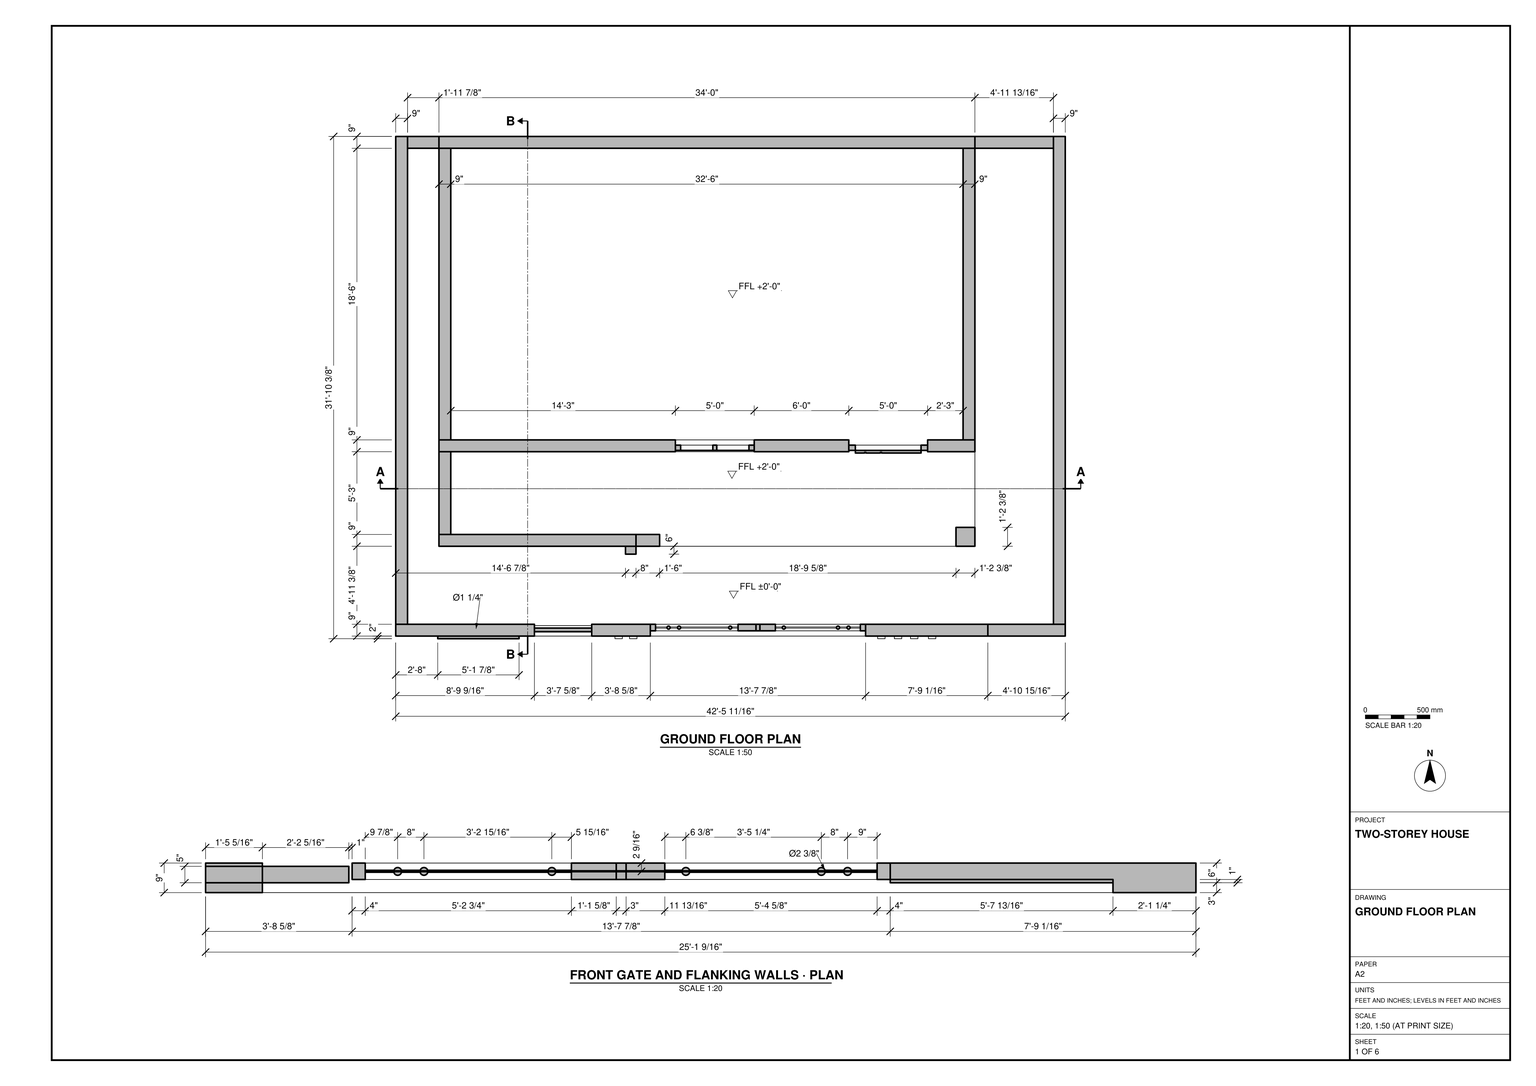
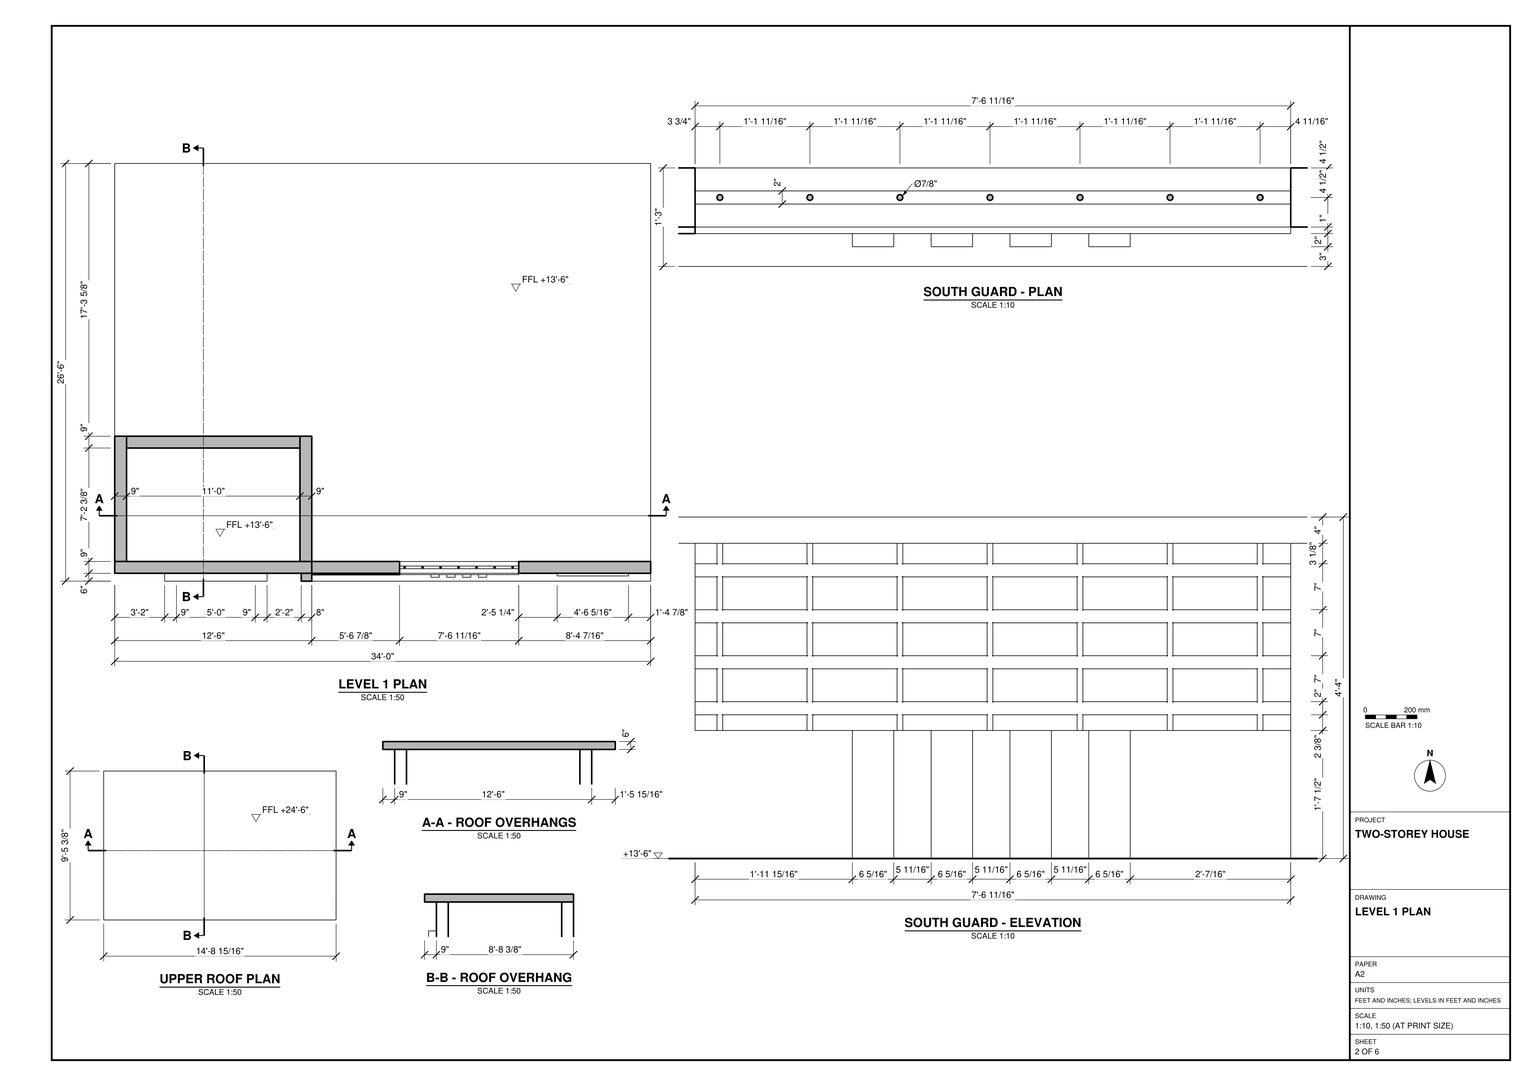
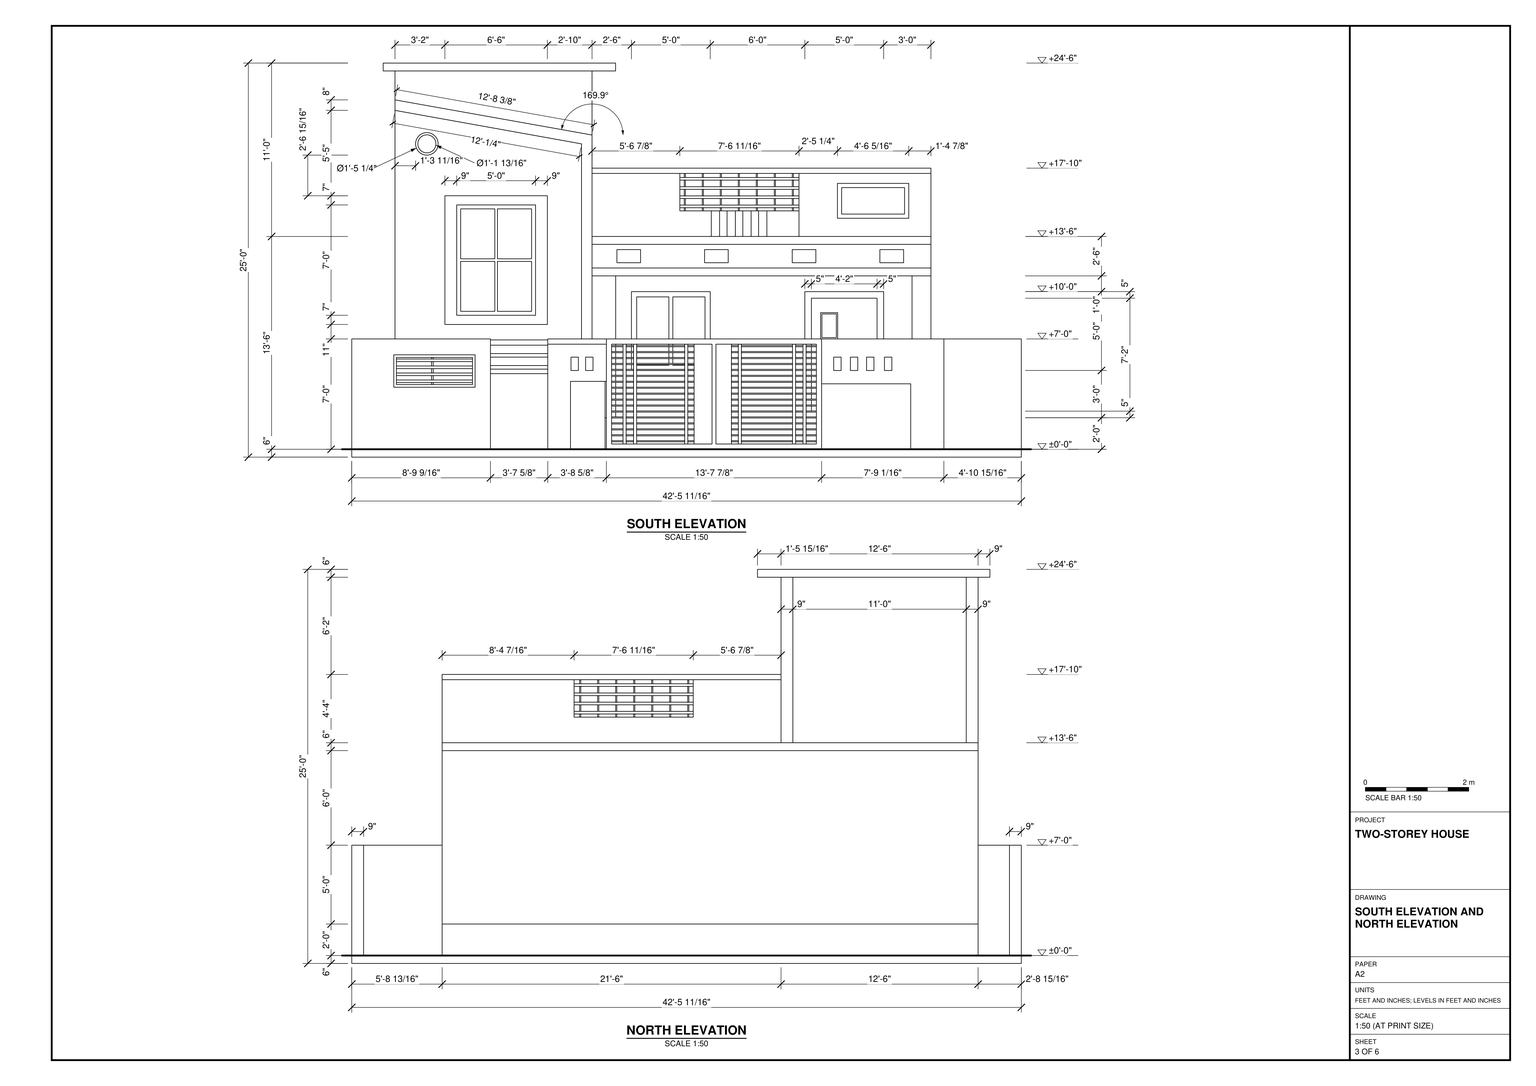
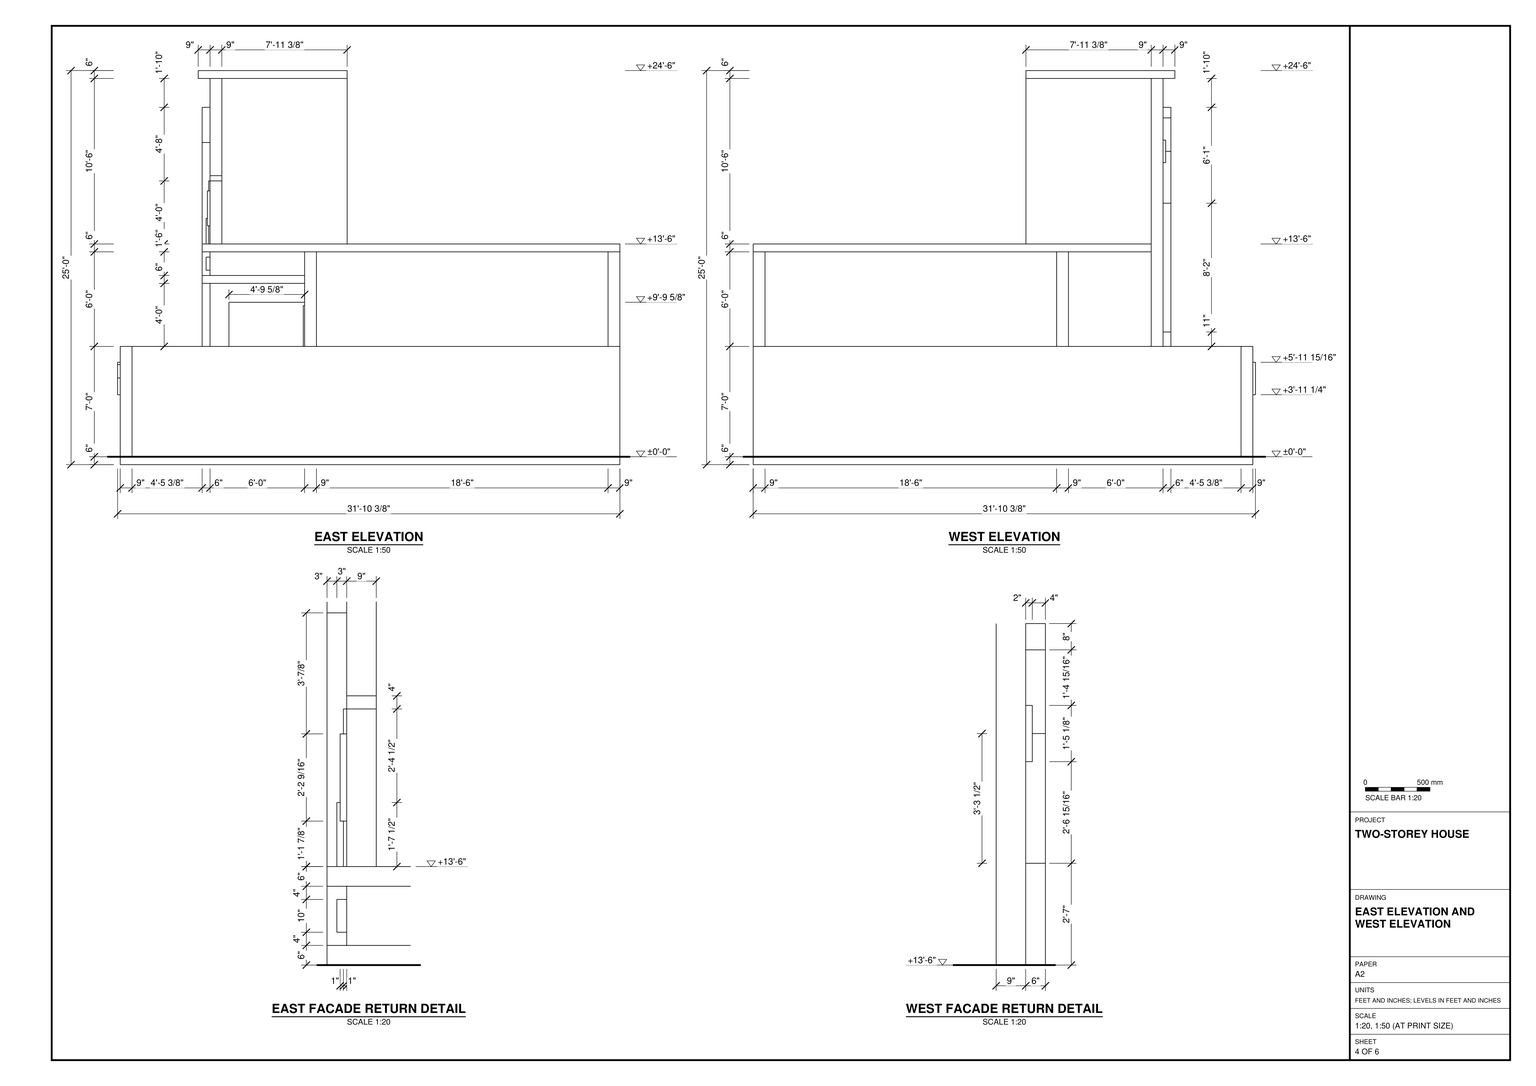
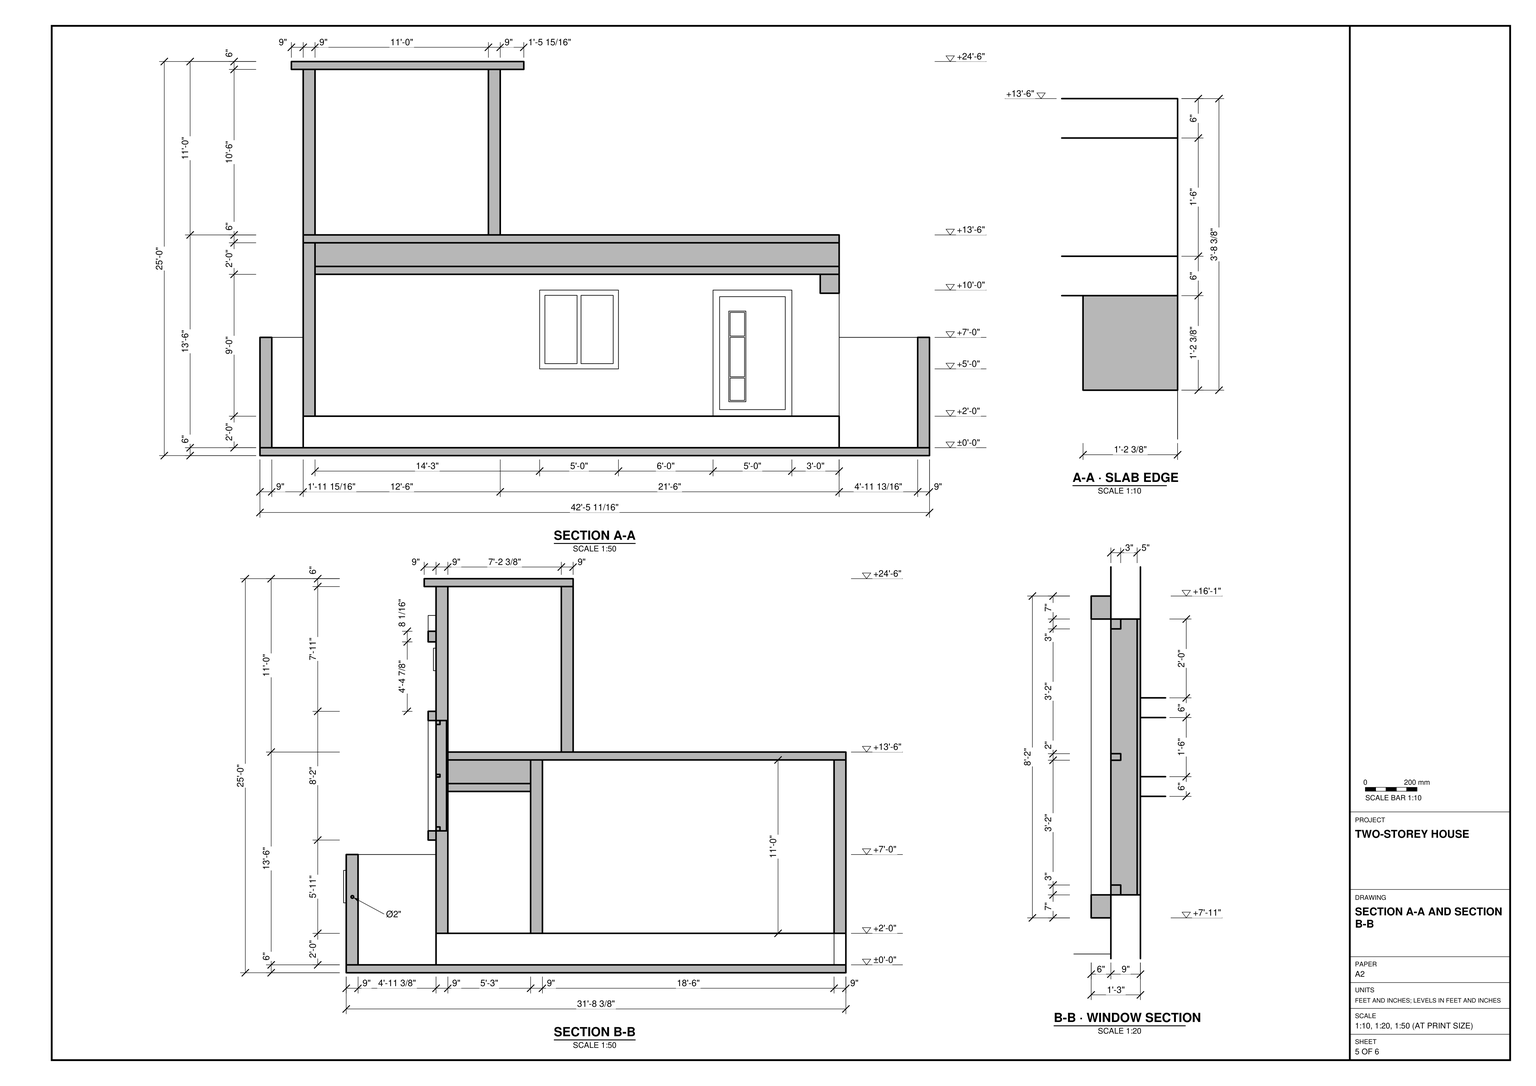
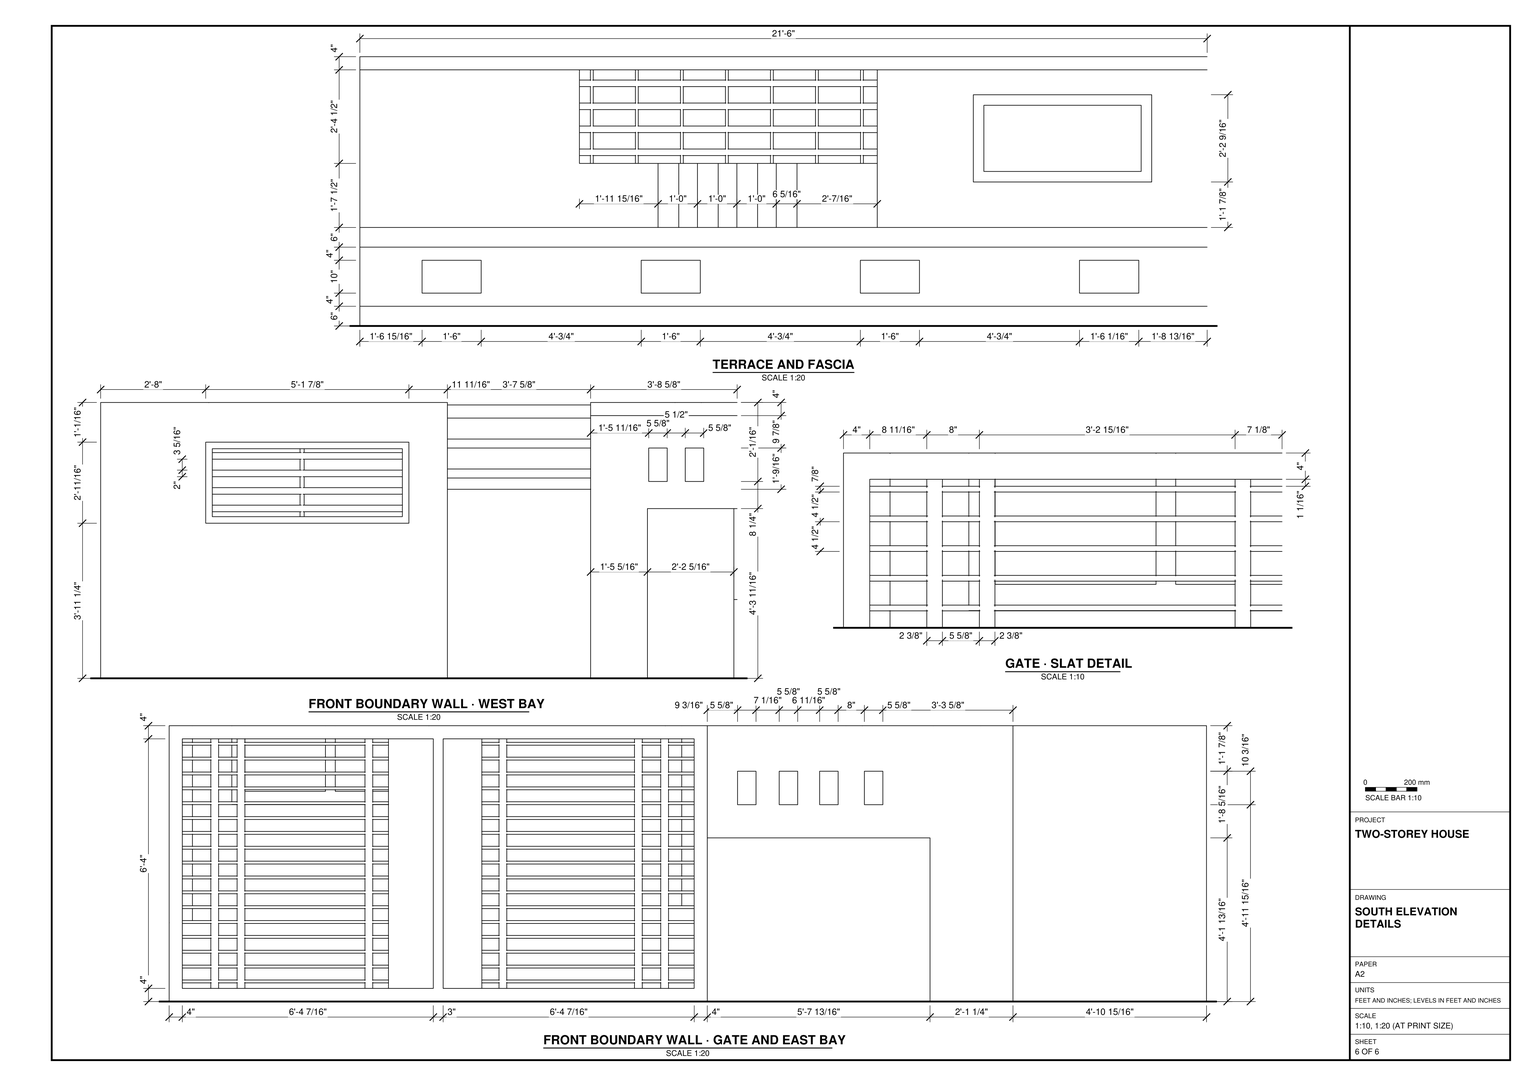
Build the house in SketchUp from task_files/diagram_01.pdf. Work in feet and inches. The overall model, including the boundary walls, is 42'-5 11/16" wide, 31'-10 3/8" deep and 25'-0" high. Use ±0'-0" as the ground datum and +13'-6" as the upper storey level. The court is at the ground datum; the porch and enclosed ground floor are raised to +2'-0".

Lay out the south boundary with its narrow pedestrian entrance, wide two-leaf gate and flanking wall panels. Set the house behind the court, with the covered porch in front of the main ground-floor space. Follow the wall thicknesses, openings and porch support positions on the plan. Model the upper slab as a broad terrace with a smaller roofed enclosure at its southwest corner. Match the tall divided window, circular detail and sloping band on the south face of this enclosure, but keep its projecting roof flat. Follow the guard detail where the open grille interrupts the solid terrace parapet.

Keep shell elements such as walls, slabs and roofs, and each furniture or joinery piece shown, in separate groups or components. Use components for repeated parts. Any decor or loose items shown may be represented by suitable library components. Save one SketchUp model as output_files/two_storey_house_with_a_gated_court_and_roof_terrace.skp.

# SketchUp Ruby script. Lengths in inches.
U = 1.inch
M = Sketchup.active_model
def pt(a) = Geom::Point3d.new(a.map { |v| v * U })
def face(e, loops, mat)
  f = e.add_face(loops[0].map { |a| pt(a) })
  loops[1..].each { |l| e.add_face(l.map { |a| pt(a) }).erase! }
  f.material = f.back_material = mat if mat
  f
end
# faces: each face lists its corners as indices into pts; further lists are holes
def faces(e, pts, list, mat = nil) = list.each { |f| face(e, (f[0].is_a?(Array) ? f : [f]).map { |l| l.map { |i| pts[i] } }, mat) }
# xy, xz, yz: faces in a plane at the given z, y or x. An outline is a flat list of corners, or four numbers for a rectangle; further outlines are holes
def ring(l) = l.size == 4 ? [[l[0], l[1]], [l[2], l[1]], [l[2], l[3]], [l[0], l[3]]] : l.each_slice(2).to_a
def flat(e, list, mat, &to3) = list.each { |f| face(e, (f[0].is_a?(Array) ? f : [f]).map { |l| ring(l).map { |u, v| to3.(u, v) } }, mat) }
def xy(e, z, list, mat = nil) = flat(e, list, mat) { |x, y| [x, y, z] }
def xz(e, y, list, mat = nil) = flat(e, list, mat) { |x, z| [x, y, z] }
def yz(e, x, list, mat = nil) = flat(e, list, mat) { |y, z| [x, y, z] }
def lines(e, pts, list) = list.each { |a, b| e.add_line(pt(pts[a]), pt(pts[b])) }
# prism: a flat outline (further loops are holes) pulled along v
def prism(e, loops, v, mat = nil)
  f = face(e, loops, mat); d = Geom::Vector3d.new(v.map { |x| x * U })
  f.pushpull(f.normal.samedirection?(d) ? d.length : -d.length)
end
def box(e, o, s, mat = nil) = prism(e, [[o, [o[0] + s[0], o[1], o[2]], [o[0] + s[0], o[1] + s[1], o[2]], [o[0], o[1] + s[1], o[2]]]], [0, 0, s[2]], mat)
def at(x, y, z, deg = 0) = Geom::Transformation.translation(pt([x, y, z])) * Geom::Transformation.rotation(ORIGIN, Z_AXIS, deg.degrees)
def axes(o, x, y, z) = Geom::Transformation.new([*x, 0, *y, 0, *z, 0, *pt(o).to_a, 1])
def part(name) = M.definitions.add(name)
# library, detail: a bought-in or finely detailed component or shape, given as its bounding box
def library(name, o, s) = part(name).tap { |d| box(d.entities, o, s) }
def detail(e, o, s) = box(e.add_group.entities, o, s)
def put(e, d, t, mat = nil) = e.add_instance(d, t).tap { |i| i.material = mat if mat }
def group(e, t, mat = nil) = e.add_group.tap { |g| g.transformation = t; g.material = mat if mat }.entities
root = M.entities
M.materials.add("[Color H08]").color = [0, 102, 102]
M.materials.add("[Color M00]").color = [255, 255, 255]
M.materials.add("[Color M02]").color = [198, 198, 198]
M.materials.add("[Color M05]").color = [114, 114, 114]
M.materials.add("[Color M07]").color = [58, 58, 58]
M.materials.add("[Color M08]").color = [30, 30, 30]
M.materials.add("[Color M09]").color = [0, 0, 0]
M.materials.add("[Translucent Glass Blue]").color = [107, 160, 255]
M.materials["[Translucent Glass Blue]"].alpha = 0.5
M.materials.add("[Wood Veneer 01]").color = [84, 49, 25]
c1 = part("Group\#29")
prism(c1.entities,[[[0,0.29,0.29],[0,0.13,0.5],[0,0.03,0.74],[0,0,1],[0,0.03,1.26],[0,0.13,1.5],[0,0.29,1.71],[0,0.5,1.87],[0,0.74,1.97],[0,1,2],[0,1.26,1.97],[0,1.5,1.87],[0,1.71,1.71],[0,1.87,1.5],[0,1.97,1.26],[0,2,1],[0,1.97,0.74],[0,1.87,0.5],[0,1.71,0.29],[0,1.5,0.13],[0,1.26,0.03],[0,1,0],[0,0.74,0.03],[0,0.5,0.13]]],[90.6875,0,0])
c2 = part("Group\#30")
prism(c2.entities,[[[0.55,0.86,0],[0.66,0.82,0],[0.75,0.75,0],[0.82,0.66,0],[0.86,0.55,0],[0.875,0.4375,0],[0.86,0.32,0],[0.82,0.22,0],[0.75,0.13,0],[0.66,0.06,0],[0.55,0.01,0],[0.4375,0,0],[0.32,0.01,0],[0.22,0.06,0],[0.13,0.13,0],[0.06,0.22,0],[0.01,0.32,0],[0,0.4375,0],[0.01,0.55,0],[0.06,0.66,0],[0.13,0.75,0],[0.22,0.82,0],[0.32,0.86,0],[0.4375,0.875,0]]],[0,0,28.5])
c3 = part("Group\#31")
box(c3.entities,[0,0,0],[6.31,2,19.5])
c4 = part("Group\#63")
prism(c4.entities,[[[57.875,0.74,0.03],[57.875,1,0],[57.875,1.26,0.03],[57.875,1.5,0.13],[57.875,1.71,0.29],[57.875,1.87,0.5],[57.875,1.97,0.74],[57.875,2,1],[57.875,1.97,1.26],[57.875,1.87,1.5],[57.875,1.71,1.71],[57.875,1.5,1.87],[57.875,1.26,1.97],[57.875,1,2],[57.875,0.74,1.97],[57.875,0.5,1.87],[57.875,0.29,1.71],[57.875,0.13,1.5],[57.875,0.03,1.26],[57.875,0,1],[57.875,0.03,0.74],[57.875,0.13,0.5],[57.875,0.29,0.29],[57.875,0.5,0.13]]],[-57.875,0,0])
c5 = part("Group\#52")
prism(c5.entities,[[[43.62,0.08,0.89],[43.62,0.25,0.58],[43.62,0.49,0.3125],[43.62,0.79,0.12],[43.62,1.14,0.01],[43.62,1.49,0],[43.62,1.84,0.08],[43.62,2.16,0.25],[43.62,2.43,0.49],[43.62,2.62,0.79],[43.62,2.72,1.14],[43.62,2.74,1.49],[43.62,2.66,1.84],[43.62,2.49,2.16],[43.62,2.25,2.43],[43.62,1.95,2.62],[43.62,1.6,2.72],[43.62,1.24,2.74],[43.62,0.89,2.66],[43.62,0.58,2.49],[43.62,0.3125,2.25],[43.62,0.12,1.95],[43.62,0.01,1.6],[43.62,0,1.24]]],[-43.62,0,0])
c6 = part("Group\#54")
prism(c6.entities,[[[155.86,0.22,0.06],[155.86,0.32,0.01],[155.86,0.4375,0],[155.86,0.55,0.01],[155.86,0.66,0.06],[155.86,0.75,0.13],[155.86,0.82,0.22],[155.86,0.86,0.32],[155.86,0.875,0.4375],[155.86,0.86,0.55],[155.86,0.82,0.66],[155.86,0.75,0.75],[155.86,0.66,0.82],[155.86,0.55,0.86],[155.86,0.4375,0.875],[155.86,0.32,0.86],[155.86,0.22,0.82],[155.86,0.13,0.75],[155.86,0.06,0.66],[155.86,0.01,0.55],[155.86,0,0.4375],[155.86,0.01,0.32],[155.86,0.06,0.22],[155.86,0.13,0.13]]],[-155.86,0,0])
c7 = part("Group\#55")
prism(c7.entities,[[[0.35,2.03,0],[0.59,2.22,0],[0.88,2.33,0],[1.1875,2.375,0],[1.49,2.33,0],[1.78,2.22,0],[2.03,2.03,0],[2.22,1.78,0],[2.33,1.49,0],[2.375,1.1875,0],[2.33,0.88,0],[2.22,0.59,0],[2.03,0.35,0],[1.78,0.16,0],[1.49,0.04,0],[1.1875,0,0],[0.88,0.04,0],[0.59,0.16,0],[0.35,0.35,0],[0.16,0.59,0],[0.04,0.88,0],[0,1.1875,0],[0.04,1.49,0],[0.16,1.78,0]]],[0,0,76])
c8 = part("Group\#58")
box(c8.entities,[0,0,0],[5.625,2,10.1875])
g1 = group(root,at(0,2,0))
box(g1,[0,0,0],[509.6875,380.37,6])
g2 = group(root,at(80.9,142.37,6))
box(g2,[-47.99,-72,0],[407.99,312,24])
g3 = group(root,at(80.9,142.37,30),"[Color M02]")
prism(g3,[[[264,9,0],[-47.99,9,0],[-47.99,9,132],[102,9,132],[360,9,132],[360,9,0],[324,9,0],[324,9,96],[264,9,96]],[[132,9,96],[132,9,36],[192,9,36],[192,9,96]]],[0,-9,0])
g4 = group(root,at(212.9,143.37,66),"[Wood Veneer 01]")
prism(g4,[[[60,4,60],[60,4,0],[0,4,0],[0,4,60]],[[28.5,4,4],[28.5,4,56],[4,4,56],[4,4,4]],[[56,4,56],[31.5,4,56],[31.5,4,4],[56,4,4]]],[0,-4,0])
g5 = group(root,at(344.9,143.37,30),"[Wood Veneer 01]")
prism(g5,[[[0,0,0],[60,0,0],[60,0,96],[0,0,96]],[[55,0,5],[5,0,5],[5,0,91],[55,0,91]]],[0,4,0])
g6 = group(root,at(349.9,141.37,35),"[Wood Veneer 01]")
xy(g6,0,[[0,0,50,2]])
xy(g6,6,[[7,0,20,0.5]])
xy(g6,7,[[8,0,19,0.5]])
xy(g6,24,[[8,0,19,0.5]])
xy(g6,25,[[8,0,19,0.5]])
xy(g6,55,[[8,0,19,0.5]])
xy(g6,56,[[8,0,19,0.5]])
xy(g6,74,[[8,0,19,0.5]])
xy(g6,75,[[7,0,20,0.5]])
xy(g6,86,[[0,0,50,2]])
xz(g6,0,[[[0,0,50,86],[7,6,20,75]],[8,7,19,24],[8,25,19,55],[8,56,19,74]])
xz(g6,0.5,[[[7,6,20,75],[8,25,19,55],[8,56,19,74],[8,7,19,24]]])
xz(g6,2,[[0,0,50,86]])
yz(g6,0,[[0,0,2,86]])
yz(g6,7,[[0,6,0.5,75]])
yz(g6,8,[[0,7,0.5,24],[0,25,0.5,55],[0,56,0.5,74]])
yz(g6,19,[[0,7,0.5,24],[0,25,0.5,55],[0,56,0.5,74]])
yz(g6,20,[[0,6,0.5,75]])
yz(g6,50,[[0,0,2,86]])
g7 = group(root,at(32.91,373.37,30))
box(g7,[0,0,0],[407.99,9,132])
g8 = group(root,at(431.9,151.37,30))
box(g8,[0,0,0],[9,222,132])
g9 = group(root,at(32.91,151.37,30))
box(g9,[0,0,0],[9,222,132])
g10 = group(root,at(32.91,142.37,162))
prism(g10,[[[407.99,240,0],[407.99,-78,0],[149.99,-78,0],[149.99,-63,0],[0,-63,0],[0,240,0]]],[0,0,6])
g11 = group(root,at(32.91,70.37,30),"[Color H08]")
xy(g11,0,[[0,0,149.99,9]])
xy(g11,78,[[46.99,0,106.99,9]])
xy(g11,162,[[46.99,0,106.99,9]])
xy(g11,264,[[0,0,149.99,9]])
xz(g11,0,[[141.99,0,149.99,0,149.99,264,0,264,0,234,141.99,208.51]])
xz(g11,0,[[[0,0,141.99,0,141.99,208.51,0,234],[46.99,78,106.99,162]]],"[Color M05]")
xz(g11,9,[[[0,0,149.99,264],[46.99,78,106.99,162]]])
yz(g11,0,[[0,0,9,264]])
yz(g11,46.99,[[0,78,9,162]])
yz(g11,106.99,[[0,78,9,162]])
yz(g11,149.99,[[0,0,9,264]])
g12 = group(root,at(182.9,70.37,30))
box(g12,[0,0,0],[18,9,108])
g13 = group(root,at(200.9,79.37,144))
prism(g13,[[[-158.99,63,0],[240,63,0],[240,-9,0],[-18,-9,0],[-18,0,0],[-158.99,0,0]]],[0,0,18])
g14 = group(root,at(200.9,79.37,138))
prism(g14,[[[-158.99,63,0],[240,63,0],[240,-15,0],[-18,-15,0],[-18,0,0],[-158.99,0,0]]],[0,0,6])
g15 = group(root,at(79.9,78.37,108))
box(g15,[0,0,0],[60,1,84])
g16 = group(root,at(70.9,64.37,101))
prism(g16,[[[78,0,0],[78,0,98],[0,0,98],[0,0,0]],[[9,0,7],[9,0,91],[69,0,91],[69,0,7]]],[0,6,0])
g17 = group(root,at(79.9,70.37,108),"[Color M09]")
prism(g17,[[[0,3,0],[0,3,84],[60,3,84],[60,3,0]],[[29,3,43],[29,3,81],[3,3,81],[3,3,43]],[[3,3,3],[29,3,3],[29,3,41],[3,3,41]],[[57,3,3],[57,3,41],[31,3,41],[31,3,3]],[[57,3,81],[31,3,81],[31,3,43],[57,3,43]]],[0,-3,0])
g18 = group(root,at(82.9,70.37,151),"[Translucent Glass Blue]")
xz(g18,0,[[0,0,26,38]])
g19 = group(root,at(110.9,70.37,151),"[Translucent Glass Blue]")
xz(g19,0,[[0,0,26,38]])
g20 = group(root,at(82.9,70.37,111),"[Translucent Glass Blue]")
xz(g20,0,[[0,0,26,38]])
g21 = group(root,at(110.9,70.37,111),"[Translucent Glass Blue]")
xz(g21,0,[[0,0,26,38]])
g22 = group(root,at(201.84,67.37,150),"[Color M05]")
box(g22,[0,0,-2],[18,3,10])
g23 = group(root,at(268.57,67.37,150),"[Color M05]")
box(g23,[0,0,-2],[18,3,10])
g24 = group(root,at(335.3,67.37,150),"[Color M05]")
box(g24,[0,0,-2],[18,3,10])
g25 = group(root,at(402.03,67.37,150),"[Color M05]")
box(g25,[0,0,-2],[18.0625,3,10])
g26 = group(root,at(182.9,70.37,168),"[Color M05]")
xy(g26,0,[[0,0,258,9]])
xy(g26,13.84,[[186.8,-2,241.11,0]])
xy(g26,17.05,[[190.01,-2,237.91,4]],"[Color M00]")
xy(g26,19.5,[[66.86,0,157.55,9]])
xy(g26,37.2,[[190.01,-2,237.91,4]],"[Color M00]")
xy(g26,40.41,[[186.8,-2,241.11,0]])
xy(g26,48,[[0,0,66.86,9],[157.55,0,258,9]])
xz(g26,-2,[[[186.8,13.84,241.11,40.41],[190.01,17.05,237.91,37.2]]],"[Color M00]")
xz(g26,0,[[[0,0,258,0,258,48,157.55,48,157.55,19.5,66.86,19.5,66.86,48,0,48],[186.8,13.84,241.11,40.41]]])
xz(g26,4,[[190.01,17.05,237.91,37.2]],"[Color M00]")
xz(g26,9,[[0,0,0,48,66.86,48,66.86,19.5,157.55,19.5,157.55,48,258,48,258,0]])
yz(g26,0,[[0,0,9,48]])
yz(g26,66.86,[[0,19.5,9,48]])
yz(g26,157.55,[[0,19.5,9,48]])
yz(g26,186.8,[[-2,13.84,0,40.41]])
yz(g26,190.01,[[-2,17.05,4,37.2]],"[Color M00]")
yz(g26,237.91,[[-2,17.05,4,37.2]],"[Color M00]")
yz(g26,241.11,[[-2,13.84,0,40.41]])
yz(g26,258,[[0,0,9,48]])
g27 = group(root,at(182.9,69.37,168),"[Color H08]")
prism(g27,[[[0,0,48],[0,0,0],[157.55,0,0],[157.55,0,19.5],[66.86,0,19.5],[66.86,0,48]]],[0,1,0])
g28 = group(root,at(182.9,70.37,216))
box(g28,[0,0,0],[258,9,4])
put(root,c1,at(249.76,73.87,189.89))
put(root,c1,at(249.76,73.87,196.89))
put(root,c1,at(249.76,73.87,203.89))
put(root,c1,at(249.76,73.87,210.89))
put(root,c2,at(253.09,74.43,187.5))
put(root,c2,at(266.8,74.43,187.5))
put(root,c2,at(280.51,74.43,187.5))
put(root,c2,at(294.22,74.43,187.5))
put(root,c2,at(307.93,74.43,187.5))
put(root,c2,at(321.63,74.43,187.5))
put(root,c2,at(335.34,74.43,187.5))
put(root,c3,at(285.7,67.37,168))
put(root,c3,at(297.7,67.37,168))
put(root,c3,at(273.7,67.37,168))
put(root,c3,at(309.7,67.37,168))
g29 = group(root,at(244.4,143.37,70),"[Translucent Glass Blue]")
xz(g29,0,[[0,0,24.5,52]])
g30 = group(root,at(216.9,143.37,70),"[Translucent Glass Blue]")
xz(g30,0,[[0,0,24.5,52]])
g31 = group(root,at(32.91,64.37,30))
prism(g31,[[[141.99,6,0],[141.99,6,208.51],[0,6,234],[0,6,242],[149.99,6,215.25],[149.99,6,0]]],[0,-6,0])
g32 = group(root,at(173.9,79.37,168),"[Color H08]")
box(g32,[0,0,0],[9,95.37,126])
g33 = group(root,at(41.91,165.74,168))
box(g33,[0,0,0],[131.99,9,126])
g34 = group(root,at(32.91,79.37,168))
box(g34,[0,0,0],[9,95.37,126])
g35 = group(root,at(32.91,70.37,294))
box(g35,[-9,-9,0],[176.93,113.37,6])
g36 = group(root,at(48.6,68.37,229.95))
xz(g36,0,[[[9.61,0,11.79,0.5625,13.75,1.67,15.35,3.25,16.5,5.18,17.1,7.35,17.125,9.61,16.5625,11.79,15.45,13.75,13.88,15.35,11.9375,16.5,9.77,17.1,7.52,17.125,5.34,16.5625,3.38,15.45,1.77,13.88,0.625,11.9375,0.02,9.77,0,7.52,0.5625,5.34,1.67,3.38,3.25,1.77,5.18,0.625,7.35,0.02],[9.4,1.7,7.59,1.72,5.86,2.2,4.3,3.12,3.04,4.41,2.15,5.98,1.7,7.73,1.72,9.53,2.2,11.27,3.12,12.82,4.41,14.09,5.98,14.97,7.73,15.42,9.53,15.41,11.27,14.92,12.82,14,14.09,12.72,14.97,11.15,15.42,9.4,15.41,7.59,14.92,5.86,14,4.3,12.72,3.04,11.15,2.15]]])
xz(g36,1,[[9.4,1.7,7.59,1.72,5.86,2.2,4.3,3.12,3.04,4.41,2.15,5.98,1.7,7.73,1.72,9.53,2.2,11.27,3.12,12.82,4.41,14.09,5.98,14.97,7.73,15.42,9.53,15.41,11.27,14.92,12.82,14,14.09,12.72,14.97,11.15,15.42,9.4,15.41,7.59,14.92,5.86,14,4.3,12.72,3.04,11.15,2.15]],"[Color H08]")
xz(g36,2,[[[9.61,0,7.35,0.02,5.18,0.625,3.25,1.77,1.67,3.38,0.5625,5.34,0,7.52,0.02,9.77,0.625,11.9375,1.77,13.88,3.38,15.45,5.34,16.5625,7.52,17.125,9.77,17.1,11.9375,16.5,13.88,15.35,15.45,13.75,16.5625,11.79,17.125,9.61,17.1,7.35,16.5,5.18,15.35,3.25,13.75,1.67,11.79,0.5625],[9.4,1.7,11.15,2.15,12.72,3.04,14,4.3,14.92,5.86,15.41,7.59,15.42,9.4,14.97,11.15,14.09,12.72,12.82,14,11.27,14.92,9.53,15.41,7.73,15.42,5.98,14.97,4.41,14.09,3.12,12.82,2.2,11.27,1.72,9.53,1.7,7.73,2.15,5.98,3.04,4.41,4.3,3.12,5.86,2.2,7.59,1.72]]])
p = [[5.18,2,0.625],[7.35,2,0.02],[7.35,0,0.02],[5.18,0,0.625],[9.61,2,0],[9.61,0,0],
  [11.79,2,0.5625],[11.79,0,0.5625],[3.25,2,1.77],[3.25,0,1.77],[13.75,2,1.67],[13.75,0,1.67],
  [7.59,0,1.72],[7.59,1,1.72],[5.86,1,2.2],[5.86,0,2.2],[9.4,0,1.7],[9.4,1,1.7],
  [11.15,0,2.15],[11.15,1,2.15],[15.35,2,3.25],[15.35,0,3.25],[7.59,2,1.72],[5.86,2,2.2],
  [9.4,2,1.7],[11.15,2,2.15],[1.67,2,3.38],[1.67,0,3.38],[4.3,1,3.12],[4.3,0,3.12],
  [12.72,0,3.04],[12.72,1,3.04],[4.3,2,3.12],[12.72,2,3.04],[14,0,4.3],[14,1,4.3],
  [14,2,4.3],[3.04,1,4.41],[3.04,0,4.41],[3.04,2,4.41],[16.5,2,5.18],[16.5,0,5.18],
  [0.5625,2,5.34],[0.5625,0,5.34],[14.92,0,5.86],[14.92,1,5.86],[14.92,2,5.86],[2.15,1,5.98],
  [2.15,0,5.98],[2.15,2,5.98],[17.1,2,7.35],[17.1,0,7.35],[0,2,7.52],[0,0,7.52],
  [15.41,0,7.59],[15.41,1,7.59],[15.41,2,7.59],[1.7,1,7.73],[1.7,0,7.73],[1.7,2,7.73],
  [17.125,2,9.61],[17.125,0,9.61],[0.02,2,9.77],[0.02,0,9.77],[15.42,0,9.4],[15.42,1,9.4],
  [15.42,2,9.4],[1.72,1,9.53],[1.72,0,9.53],[1.72,2,9.53],[14.97,0,11.15],[14.97,1,11.15],
  [14.97,2,11.15],[2.2,1,11.27],[2.2,0,11.27],[2.2,2,11.27],[16.5625,2,11.79],[16.5625,0,11.79],
  [0.625,2,11.9375],[0.625,0,11.9375],[14.09,0,12.72],[14.09,1,12.72],[14.09,2,12.72],[3.12,1,12.82],
  [3.12,0,12.82],[3.12,2,12.82],[15.45,2,13.75],[15.45,0,13.75],[1.77,2,13.88],[1.77,0,13.88],
  [12.82,0,14],[12.82,1,14],[12.82,2,14],[4.41,1,14.09],[4.41,0,14.09],[4.41,2,14.09],
  [13.88,2,15.35],[13.88,0,15.35],[3.38,2,15.45],[3.38,0,15.45],[11.27,0,14.92],[11.27,1,14.92],
  [11.27,2,14.92],[5.98,1,14.97],[5.98,0,14.97],[5.98,2,14.97],[9.53,0,15.41],[9.53,1,15.41],
  [9.53,2,15.41],[7.73,1,15.42],[7.73,0,15.42],[7.73,2,15.42],[11.9375,2,16.5],[11.9375,0,16.5],
  [5.34,2,16.5625],[5.34,0,16.5625],[9.77,2,17.1],[9.77,0,17.1],[7.52,2,17.125],[7.52,0,17.125]]
faces(g36,p,[[0,1,2,3],[1,4,5,2],[4,6,7,5],[8,0,3,9],[6,10,11,7],[12,13,14,15],[16,17,13,12],[18,19,17,16],
  [10,20,21,11],[22,23,14,13],[24,22,13,17],[25,24,17,19],[26,8,9,27],[15,14,28,29],[30,31,19,18],[23,32,28,14],
  [33,25,19,31],[34,35,31,30],[36,33,31,35],[29,28,37,38],[32,39,37,28],[20,40,41,21],[42,26,27,43],[44,45,35,34],
  [46,36,35,45],[38,37,47,48],[39,49,47,37],[40,50,51,41],[52,42,43,53],[54,55,45,44],[56,46,45,55],[48,47,57,58],
  [49,59,57,47],[50,60,61,51],[62,52,53,63],[64,65,55,54],[66,56,55,65],[58,57,67,68],[59,69,67,57],[70,71,65,64],
  [72,66,65,71],[68,67,73,74],[69,75,73,67],[60,76,77,61],[78,62,63,79],[80,81,71,70],[82,72,71,81],[74,73,83,84],
  [75,85,83,73],[76,86,87,77],[88,78,79,89],[90,91,81,80],[92,82,81,91],[84,83,93,94],[85,95,93,83],[86,96,97,87],
  [98,88,89,99],[100,101,91,90],[102,92,91,101],[94,93,103,104],[95,105,103,93],[106,107,101,100],[108,102,101,107],[104,103,109,110],
  [105,111,109,103],[110,109,107,106],[96,112,113,97],[111,108,107,109],[114,98,99,115],[112,116,117,113],[118,114,115,119],[116,118,119,117]])
g37 = group(root,at(426.5,70.37,30))
prism(g37,[[[0,14.4,0],[0,0,0],[0,0,108],[0,72,108],[0,72,93.6],[0,14.4,93.6]]],[14.4,0,0])
g38 = group(root,at(32.91,79.37,30))
box(g38,[0,0,0],[9,63,132])
g39 = group(root,at(450.76,2,6),"[Color H08]")
box(g39,[0,0,0],[58.93,9,84])
g40 = group(root,at(357.68,2,6),"[Color M05]")
xy(g40,0,[[67.83,0,67.83,4,0,4,0,9,93.08,9,93.08,0]])
xy(g40,49.84,[[0,0,67.83,4]])
xy(g40,84,[[0,0,93.08,9]])
xz(g40,0,[[67.83,0,93.08,0,93.08,84,0,84,0,49.84,67.83,49.84]])
xz(g40,4,[[0,0,67.83,49.84]])
xz(g40,9,[[0,0,93.08,84]])
yz(g40,0,[[4,0,4,49.84,0,49.84,0,84,9,84,9,0]])
yz(g40,67.83,[[0,0,4,49.84]])
yz(g40,93.08,[[0,0,9,84]])
g41 = group(root,at(357.68,5,6),"[Color H08]")
box(g41,[0,0,0],[67.83,1,49.84])
g42 = group(root,at(-24,2,6),"[Color M02]")
prism(g42,[[[24,0,0],[129.58,0,0],[129.58,0,84],[24,0,84]],[[57.99,0,49.23],[57.99,0,69.92],[115.87,0,69.92],[115.87,0,49.23]]],[0,9,0])
put(root,c4,at(33.99,5.67,72.73))
put(root,c4,at(33.99,5.67,67.4))
put(root,c4,at(33.99,5.67,62.07))
g43 = group(root,at(57.99,5.67,56.73))
prism(g43,[[[57.875,0.74,0.03],[57.875,1,0],[57.875,1.26,0.03],[57.875,1.5,0.13],[57.875,1.71,0.29],[57.875,1.87,0.5],[57.875,1.97,0.74],[57.875,2,1],[57.875,1.97,1.26],[57.875,1.87,1.5],[57.875,1.71,1.71],[57.875,1.5,1.87],[57.875,1.26,1.97],[57.875,1,2],[57.875,0.74,1.97],[57.875,0.5,1.87],[57.875,0.29,1.71],[57.875,0.13,1.5],[57.875,0.03,1.26],[57.875,0,1],[57.875,0.03,0.74],[57.875,0.13,0.5],[57.875,0.29,0.29],[57.875,0.5,0.13]]],[-81.875,0,0])
g44 = group(root,at(60.71,6.3125,55.23))
prism(g44,[[[0.625,1.25,0],[0.79,1.23,0],[0.9375,1.17,0],[1.07,1.07,0],[1.17,0.9375,0],[1.23,0.79,0],[1.25,0.625,0],[1.23,0.46,0],[1.17,0.3125,0],[1.07,0.18,0],[0.9375,0.08,0],[0.79,0.02,0],[0.625,0,0],[0.46,0.02,0],[0.3125,0.08,0],[0.18,0.18,0],[0.08,0.3125,0],[0.02,0.46,0],[0,0.625,0],[0.02,0.79,0],[0.08,0.9375,0],[0.18,1.07,0],[0.3125,1.17,0],[0.46,1.23,0]]],[0,0,20.6875])
g45 = group(root,at(105.58,2,6),"[Color H08]")
box(g45,[0,3,0],[87.23,5,57.57])
g46 = group(root,at(149.2,2,6),"[Color M05]")
prism(g46,[[[0,9,80],[44.62,9,80],[44.62,9,51.69],[17.3,9,51.69],[17.3,9,0],[0,9,0]]],[0,-9,0])
g47 = group(root,at(149.2,2,86))
box(g47,[0,0,0],[44.62,9,4])
g48 = group(root,at(105.58,4.33,85.25))
prism(g48,[[[0,2,0],[0,1.48,0.07],[0,1,0.27],[0,0.59,0.59],[0,0.27,1],[0,0.07,1.48],[0,0,2],[0,0.07,2.52],[0,0.27,3],[0,0.59,3.41],[0,1,3.73],[0,1.48,3.93],[0,2,4],[0,2.52,3.93],[0,3,3.73],[0,3.41,3.41],[0,3.73,3],[0,3.93,2.52],[0,4,2],[0,3.93,1.48],[0,3.73,1],[0,3.41,0.59],[0,3,0.27],[0,2.52,0.07]]],[43.62,0,0])
put(root,c5,at(105.58,5.39,76.125))
put(root,c5,at(105.58,5.39,67))
g49 = group(root,at(193.8125,6,6),"[Color M08]")
prism(g49,[[[163.86,5,84],[163.86,5,0],[0,5,0],[0,5,84]],[[159.86,5,80],[83.43,5,80],[83.43,5,4],[159.86,5,4]],[[80.43,5,4],[80.43,5,80],[4,5,80],[4,5,4]]],[0,-5,0])
put(root,c6,at(197.8125,8.0625,84.06),"[Color M08]")
put(root,c6,at(197.8125,8.0625,79.53),"[Color M08]")
put(root,c6,at(197.8125,8.0625,75.01),"[Color M08]")
put(root,c6,at(197.8125,8.0625,70.49),"[Color M08]")
put(root,c6,at(197.8125,8.0625,65.96),"[Color M08]")
put(root,c6,at(197.8125,8.0625,61.44),"[Color M08]")
put(root,c6,at(197.8125,8.0625,56.92),"[Color M08]")
put(root,c6,at(197.8125,8.0625,52.39),"[Color M08]")
put(root,c6,at(197.8125,8.0625,47.87),"[Color M08]")
put(root,c6,at(197.8125,8.0625,43.35),"[Color M08]")
put(root,c6,at(197.8125,8.0625,38.82),"[Color M08]")
put(root,c6,at(197.8125,8.0625,34.3),"[Color M08]")
put(root,c6,at(197.8125,8.0625,29.78),"[Color M08]")
put(root,c6,at(197.8125,8.0625,25.25),"[Color M08]")
put(root,c6,at(197.8125,8.0625,20.73),"[Color M08]")
put(root,c6,at(197.8125,8.0625,16.21),"[Color M08]")
put(root,c6,at(197.8125,8.0625,11.68),"[Color M08]")
put(root,c7,at(206.5,7.27,10),"[Color M08]")
put(root,c7,at(214.5,7.27,10),"[Color M08]")
put(root,c7,at(343.5,7.27,10),"[Color M08]")
put(root,c7,at(335.5,7.27,10),"[Color M08]")
g50 = group(root,at(260.59,6,10),"[Color M07]")
box(g50,[0,0,0],[13.65,5,76])
g51 = group(root,at(277.24,6,10),"[Color M07]")
box(g51,[0,0,0],[11.79,5,76])
put(root,c7,at(253.4375,7.27,10),"[Color M08]")
put(root,c7,at(294.25,7.27,10),"[Color M08]")
put(root,c8,at(166.89,0,65.95))
put(root,c8,at(178.01,0,65.95))
put(root,c8,at(366.89,0,65.95))
put(root,c8,at(379.58,0,65.95))
put(root,c8,at(391.89,0,65.95))
put(root,c8,at(405.51,0,65.95))
g52 = group(root,at(500.6875,11,6))
box(g52,[0,0,0],[9,371.37,84])
g53 = group(root,at(440.9,373.37,6))
box(g53,[0,0,0],[59.79,9,84])
g54 = group(root,at(0,11,6))
box(g54,[0,0,0],[9,371.37,84])
g55 = group(root,at(9,373.37,6))
box(g55,[0,0,0],[23.91,9,84])
g56 = group(root,at(31.99,0,53.23),"[Color M05]")
prism(g56,[[[0,2,0],[0,2,24.6875],[61.875,2,24.6875],[61.875,2,0]],[[2,2,2],[59.875,2,2],[59.875,2,22.6875],[2,2,22.6875]]],[0,-2,0])
